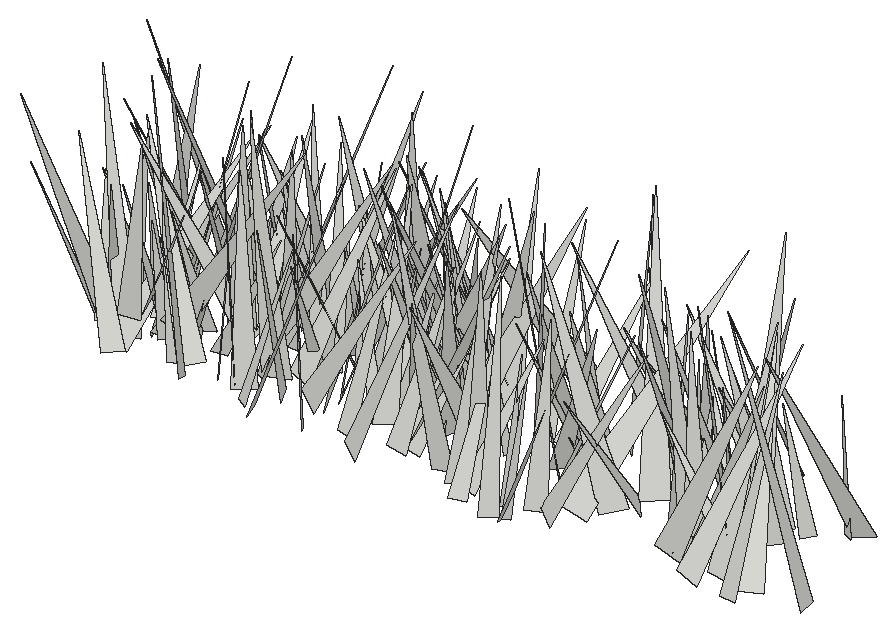
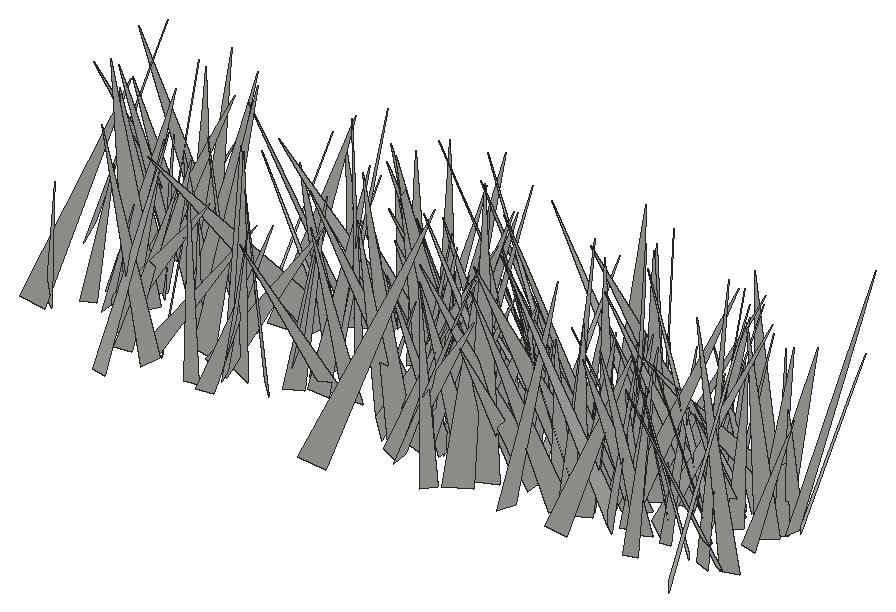
# SketchUp Ruby script. Lengths in inches.
U = 1.inch
M = Sketchup.active_model
def pt(a) = Geom::Point3d.new(a.map { |v| v * U })
def face(e, loops, mat)
  f = e.add_face(loops[0].map { |a| pt(a) })
  loops[1..].each { |l| e.add_face(l.map { |a| pt(a) }).erase! }
  f.material = f.back_material = mat if mat
  f
end
# faces: each face lists its corners as indices into pts; further lists are holes
def faces(e, pts, list, mat = nil) = list.each { |f| face(e, (f[0].is_a?(Array) ? f : [f]).map { |l| l.map { |i| pts[i] } }, mat) }
# xy, xz, yz: faces in a plane at the given z, y or x. An outline is a flat list of corners, or four numbers for a rectangle; further outlines are holes
def ring(l) = l.size == 4 ? [[l[0], l[1]], [l[2], l[1]], [l[2], l[3]], [l[0], l[3]]] : l.each_slice(2).to_a
def flat(e, list, mat, &to3) = list.each { |f| face(e, (f[0].is_a?(Array) ? f : [f]).map { |l| ring(l).map { |u, v| to3.(u, v) } }, mat) }
def xy(e, z, list, mat = nil) = flat(e, list, mat) { |x, y| [x, y, z] }
def xz(e, y, list, mat = nil) = flat(e, list, mat) { |x, z| [x, y, z] }
def yz(e, x, list, mat = nil) = flat(e, list, mat) { |y, z| [x, y, z] }
def lines(e, pts, list) = list.each { |a, b| e.add_line(pt(pts[a]), pt(pts[b])) }
# prism: a flat outline (further loops are holes) pulled along v
def prism(e, loops, v, mat = nil)
  f = face(e, loops, mat); d = Geom::Vector3d.new(v.map { |x| x * U })
  f.pushpull(f.normal.samedirection?(d) ? d.length : -d.length)
end
def box(e, o, s, mat = nil) = prism(e, [[o, [o[0] + s[0], o[1], o[2]], [o[0] + s[0], o[1] + s[1], o[2]], [o[0], o[1] + s[1], o[2]]]], [0, 0, s[2]], mat)
def at(x, y, z, deg = 0) = Geom::Transformation.translation(pt([x, y, z])) * Geom::Transformation.rotation(ORIGIN, Z_AXIS, deg.degrees)
def axes(o, x, y, z) = Geom::Transformation.new([*x, 0, *y, 0, *z, 0, *pt(o).to_a, 1])
def part(name) = M.definitions.add(name)
# library, detail: a bought-in or finely detailed component or shape, given as its bounding box
def library(name, o, s) = part(name).tap { |d| box(d.entities, o, s) }
def detail(e, o, s) = box(e.add_group.entities, o, s)
def put(e, d, t, mat = nil) = e.add_instance(d, t).tap { |i| i.material = mat if mat }
def group(e, t, mat = nil) = e.add_group.tap { |g| g.transformation = t; g.material = mat if mat }.entities
root = M.entities
c1 = part("fur_instance\#9")
p = [[0.8125,0,1.79],[0.67,-0.02,1.48],[0,-0.11,0],[0,0.11,0]]
faces(c1.entities,p,[[0,1,2,3]])
put(root,c1,axes([95.93,447.23,-27.1],[-3.80527,0.70423,0.62745],[0.3357,3.44844,-1.83447],[0.88144,1.72686,3.40746]))
put(root,c1,axes([97.41,448.625,-27.1],[3.70489,5.29932,0.63458],[5.07029,-3.25343,-2.43293],[1.66665,-1.88258,5.99082]))
put(root,c1,axes([95.1,446.8125,-27.1],[-5.93651,2.05948,0.4431],[1.83167,5.70073,-1.95618],[1.04056,1.71471,5.97135]))
put(root,c1,axes([96.62,448.84,-27.1],[-2.20726,4.7722,2.01563],[5.04733,2.47451,-0.33147],[1.16667,-1.67676,5.24748]))
put(root,c1,axes([78.89,450.2,-27.1],[-4.44854,-2.43941,1.67916],[-2.34276,4.75236,0.69742],[1.81157,0.15557,5.02532]))
put(root,c1,axes([100.51,452.55,-27.1],[-3.99829,-3.957,0.07334],[-3.50173,3.58563,2.55553],[1.84422,-1.77059,5.01133]))
put(root,c1,axes([90.21,449.16,-27.1],[-1.59145,-6.67923,2.98055],[-7.18236,0.85085,-1.92829],[-1.38185,3.26993,6.58988]))
put(root,c1,axes([68.83,449.93,-27.1],[3.92094,-4.8226,1.73149],[-5.06492,-3.97791,0.39007],[-0.77596,1.59628,6.20315]))
put(root,c1,axes([81.86,448.05,-27.1],[-4.19914,-2.372,1.71601],[-2.90919,3.71707,-1.98087],[0.32817,2.60017,4.39719]))
put(root,c1,axes([69.15,448.31,-27.1],[-3.00084,5.06154,0.45444],[5.0055,2.85272,1.2797],[-0.87785,-1.03611,5.74339]))
put(root,c1,axes([65.8125,451.81,-27.1],[-7.05336,-2.15617,1.71578],[-1.62887,7.06566,2.18314],[2.22256,-1.66441,7.04506]))
put(root,c1,axes([78.5625,447.95,-27.1],[6.55777,3.05775,0.67545],[3.00333,-6.58518,0.65252],[-0.88663,0.30968,7.20614]))
put(root,c1,axes([85.25,447.75,-27.1],[4.54632,6.46757,0.61256],[6.48609,-4.47646,-0.87508],[0.36794,-1.0028,7.85702]))
put(root,c1,axes([104.68,449.58,-27.1],[2.05152,-6.6713,2.37008],[-6.64568,-0.96384,3.03943],[2.44098,2.98279,6.28306]))
put(root,c1,axes([95.06,448.26,-27.1],[-3.85021,0.78609,0.9669],[0.45373,3.80886,-1.28983],[1.16059,1.11875,3.71193]))
put(root,c1,axes([74.96,449.76,-27.1],[2.81827,1.89164,1.24112],[2.11841,-2.90244,-0.38665],[-0.79437,-1.02901,3.37216]))
put(root,c1,axes([65.68,451.29,-27.1],[-3.97352,-3.33663,0.47318],[-3.25036,3.98768,0.8243],[0.89005,-0.33346,5.12275]))
put(root,c1,axes([75.72,450.125,-27.1],[4.83002,3.67653,3.08875],[4.26917,-5.29337,-0.3752],[-2.19806,-2.20219,6.05848]))
put(root,c1,axes([76.89,449.51,-27.1],[3.45962,-4.50001,2.91683],[-5.02174,-3.93643,-0.1168],[-1.88153,2.2319,5.67498]))
put(root,c1,axes([77.69,448.28,-27.1],[2.30646,3.84948,0.31393],[3.83736,-2.32546,0.32205],[-0.43787,-0.10267,4.47599]))
put(root,c1,axes([92.46,448.33,-27.1],[0.05703,4.78722,0.58826],[4.57544,0.13244,-1.52137],[1.52606,-0.57598,4.5394]))
put(root,c1,axes([91.9375,449.9,-27.1],[5.0258,-2.8928,2.35137],[-3.11716,-5.42578,-0.01254],[-2.04464,1.16127,5.79886]))
put(root,c1,axes([92.71,447.29,-27.1],[-4.05374,2.9207,0.15477],[2.65047,3.78022,-1.91631],[1.23673,1.47198,4.61422]))
put(root,c1,axes([108.58,450.4375,-27.1],[-4.58076,1.47717,0.18742],[1.47131,4.39705,1.30451],[-0.22897,-1.29786,4.63288]))
put(root,c1,axes([110.08,447.79,-27.1],[1.80185,5.93958,0.37976],[5.89361,-1.83593,0.75111],[-0.82954,-0.14229,6.16126]))
put(root,c1,axes([89.45,452.92,-27.1],[5.03177,-2.92165,1.14225],[-2.20313,-4.82824,-2.64459],[-2.23316,-1.81978,5.18275]))
put(root,c1,axes([113.78,449.7,-27.1],[-7.70081,-2.50661,0.76749],[-2.60656,7.57519,-1.4131],[0.27927,1.58364,7.97425]))
put(root,c1,axes([86.01,452.38,-27.1],[5.48383,-1.63022,0.30334],[-1.45467,-5.23263,-1.82362],[-0.79597,-1.66854,5.42259]))
put(root,c1,axes([80.25,450.53,-27.1],[3.77376,6.10396,1.49671],[5.76595,-2.66802,-3.65722],[2.50047,-3.05991,6.17449]))
put(root,c1,axes([72.33,449.4,-27.1],[-0.0394,4.36961,1.02441],[4.32756,-0.23455,1.1669],[-1.18959,-0.99797,4.2111]))
put(root,c1,axes([70.46,451.1,-27.1],[2.53184,-2.74895,1.13947],[-2.76231,-2.72751,-0.44237],[-1.1067,0.51894,3.71097]))
put(root,c1,axes([88.15,452.46,-27.1],[6.15158,-3.29467,0.71793],[-3.15743,-6.15236,-1.17953],[-1.18361,-0.7112,6.87789]))
put(root,c1,axes([69.88,451.81,-27.1],[-4.44345,-1.97155,1.25823],[-1.71315,4.58269,1.13072],[1.59225,-0.57131,4.72787]))
put(root,c1,axes([87,449.35,-27.1],[0.12132,5.40428,1.16344],[5.42728,0.10479,-1.05269],[1.05091,-1.16504,5.30215]))
put(root,c1,axes([105.55,450.54,-27.1],[-7.11208,1.53537,2.26223],[1.65379,7.4363,0.15223],[2.17716,-0.6331,7.27433]))
put(root,c1,axes([73.58,448.48,-27.1],[-7.24108,-2.76695,1.69952],[-3.23599,6.49389,-3.21487],[0.2698,3.62643,7.05364]))
put(root,c1,axes([105.69,450.78,-27.1],[3.10657,-5.20372,2.6425],[-5.63717,-3.45056,-0.16782],[-1.51121,2.17421,6.05816]))
put(root,c1,axes([83.98,449.01,-27.1],[1.01663,5.56132,0.68679],[5.60282,-1.02017,-0.03274],[-0.09106,-0.68151,5.65338]))
put(root,c1,axes([68.67,451.19,-27.1],[4.5818,0.64032,0.1617],[0.65902,-4.5067,-0.82732],[-0.04299,-0.84188,4.55176]))
put(root,c1,axes([107.08,448.19,-27.1],[1.06363,7.1406,0.14161],[6.98782,-1.01087,-1.51263],[1.47601,-0.35985,7.05914]))
put(root,c1,axes([105.9,450.67,-27.1],[5.04993,-3.13211,0.88061],[-3.25342,-4.87587,1.31476],[-0.02926,1.58216,5.79512]))
put(root,c1,axes([95.79,446.95,-27.1],[6.81061,4.1437,0.72104],[3.52808,-6.3754,3.31382],[-2.28972,2.50169,7.25074]))
put(root,c1,axes([66.07,452.39,-27.1],[4.73789,-1.18845,0.72275],[-0.9672,-4.65874,-1.32025],[-0.99966,-1.12521,4.70287]))
put(root,c1,axes([91.59,448.7,-27.1],[-6.63675,3.07759,1.929],[2.57186,6.8191,-2.03087],[2.56478,1.12578,7.02806]))
put(root,c1,axes([77.43,451.46,-27.1],[-2.10134,6.53759,3.4605],[7.38552,2.05442,0.60354],[0.41142,-3.48856,6.84043]))
put(root,c1,axes([81.06,451.06,-27.1],[7.00496,3.81978,0.96353],[3.93839,-6.83549,-1.53416],[-0.09034,-1.80938,7.82984]))
put(root,c1,axes([73.15,449.84,-27.1],[-5.62336,3.63446,0.06059],[3.63174,5.6129,0.37548],[-0.15301,-0.3482,6.6851]))
put(root,c1,axes([108.1,450.74,-27.1],[-5.99226,-3.56649,1.99916],[-3.93709,5.99,-1.11487],[1.10264,2.00593,6.88361]))
put(root,c1,axes([99.76,451.31,-27.1],[-4.16416,5.80884,2.0419],[6.1268,3.66414,2.07088],[-0.6118,-2.84317,6.84063]))
put(root,c1,axes([103.8,453.76,-27.1],[-0.44109,-6.89492,0.21564],[-6.89758,0.44393,0.08524],[0.09888,0.20974,6.90849]))
put(root,c1,axes([87.5,450.59,-27.1],[6.84085,-1.05323,0.60817],[-1.14548,-6.7472,1.19982],[-0.40871,1.28156,6.81667]))
put(root,c1,axes([108.29,449.29,-27.1],[1.00933,7.00307,0.82634],[7.04916,-1.02422,0.06983],[-0.18746,-0.80782,7.07509]))
put(root,c1,axes([87.49,449.76,-27.1],[-0.99691,5.86129,1.26655],[5.41282,1.43213,-2.36709],[2.58075,-0.73958,5.45394]))
put(root,c1,axes([105.18,451.03,-27.1],[2.53545,-3.02814,1.98338],[-3.53036,-2.60371,0.53779],[-0.80002,1.89288,3.91266]))
put(root,c1,axes([108.45,451.85,-27.1],[-2.5015,-6.23633,1.72664],[-6.18785,1.76379,-2.59425],[-1.89304,2.47545,6.19832]))
put(root,c1,axes([110.48,449.07,-27.1],[-3.69849,5.78351,0.10997],[5.76561,3.69627,-0.48502],[0.46777,0.16892,6.84781]))
put(root,c1,axes([87.125,453.27,-27.1],[-0.56263,-5.96411,0.83016],[-5.9756,0.45013,-0.816],[-0.74291,0.89616,5.93475]))
put(root,c1,axes([78.87,453.23,-27.1],[0.77798,-4.23548,0.16889],[-4.23878,-0.77834,0.00619],[-0.02442,0.16723,4.30633]))
put(root,c1,axes([84.37,451.11,-27.1],[-3.97928,1.73175,0.54979],[1.73454,4.01483,-0.09183],[0.54094,-0.13447,4.3388]))
put(root,c1,axes([95.91,451.54,-27.1],[5.05169,2.87341,0.23488],[2.86098,-4.93803,-1.1233],[0.35552,-1.09113,5.70213]))
put(root,c1,axes([73.53,451.65,-27.1],[3.09859,-2.8989,0.71648],[-2.92503,-2.73871,1.56906],[0.60101,1.61681,3.94246]))
put(root,c1,axes([95.61,454.26,-27.1],[-4.40501,-3.46188,0.56585],[-3.18391,4.32713,1.68747],[1.47225,-1.00011,5.34239]))
put(root,c1,axes([70.34,451.16,-27.1],[5.69226,-5.26322,0.96159],[-5.00885,-4.7486,3.65927],[1.88086,3.28288,6.8347]))
put(root,c1,axes([71.4,452.86,-27.1],[-5.49942,-3.45806,0.94275],[-3.51329,5.5426,-0.16378],[0.70973,0.64178,6.49422]))
put(root,c1,axes([74.0625,453.6875,-27.1],[-7.08449,-0.21202,0.14595],[-0.16992,6.87165,1.73429],[0.19334,-1.72965,6.8722]))
put(root,c1,axes([104.59,449.875,-27.1],[3.23969,5.31398,1.47982],[4.81259,-3.56155,2.25346],[-2.69577,0.02794,5.80137]))
put(root,c1,axes([95.23,452.43,-27.1],[-5.96506,-5.04673,2.13711],[-5.35643,6.03696,-0.69462],[1.15994,1.92465,7.7826]))
put(root,c1,axes([66.67,450.65,-27.1],[-4.24883,1.88722,0.42776],[1.75815,4.19597,-1.04876],[0.80838,0.79335,4.52927]))
put(root,c1,axes([80.23,454.59,-27.1],[-3.47678,-4.99975,0.07246],[-4.93171,3.44331,0.95532],[0.82523,-0.48669,6.01439]))
put(root,c1,axes([87.87,451.76,-27.1],[1.06055,3.50039,1.15885],[3.68372,-1.05849,-0.17402],[-0.16095,-1.16074,3.65339]))
put(root,c1,axes([79.46,452.22,-27.1],[1.72384,-3.5656,0.8716],[-3.29525,-1.07913,2.10276],[1.61693,1.60212,3.35612]))
put(root,c1,axes([71.69,453.13,-27.1],[0.72019,-3.80208,0.86926],[-3.795,-0.88705,-0.73566],[-0.89965,0.69817,3.79912]))
put(root,c1,axes([106.7,452.5,-27.1],[-3.07228,-3.20464,1.70758],[-3.41257,3.31254,0.07678],[1.24093,1.17551,4.43878]))
put(root,c1,axes([94.75,453.05,-27.1],[4.6953,-3.04636,0.27903],[-3.0591,-4.67738,0.40996],[-0.01004,0.49581,5.58194]))
put(root,c1,axes([68.43,453.28,-27.1],[3.6116,-2.54944,1.03868],[-2.46348,-3.75778,-0.65768],[-1.22872,0.0404,4.37159]))
put(root,c1,axes([68.17,450.66,-27.1],[-6.64184,2.29308,0.28161],[2.23011,6.58737,-1.04152],[0.60342,0.8944,6.94892]))
put(root,c1,axes([66.43,453.1,-27.1],[2.75053,-5.09352,1.52718],[-5.31748,-2.64324,0.76119],[-0.02665,1.70616,5.73847]))
put(root,c1,axes([86.78,452.53,-27.1],[-3.90024,1.94852,0.94584],[2.05782,3.9414,0.36592],[0.67579,-0.75618,4.3445]))
put(root,c1,axes([68.76,448.98,-27.1],[-3.50989,5.55769,0.51718],[4.45011,3.15505,-3.70364],[3.36927,1.62248,5.4305]))
put(root,c1,axes([103.18,453.01,-27.1],[-1.62958,-3.15436,1.09529],[-3.33909,1.53504,-0.54711],[-0.01197,1.22427,3.50802]))
put(root,c1,axes([73.36,453.7,-27.1],[4.72126,-4.87179,1.88096],[-5.03873,-4.91595,-0.08523],[-1.37242,1.28908,6.78361]))
put(root,c1,axes([75.08,453.34,-27.1],[4.55418,4.59674,3.34406],[5.23121,-5.06575,-0.16086],[-2.22422,-2.50228,6.46875]))
put(root,c1,axes([92.86,453.63,-27.1],[6.58164,2.52237,2.667],[2.99732,-6.85363,-0.91486],[-2.11926,-1.85972,6.9888]))
put(root,c1,axes([108.49,453.9,-27.1],[-3.08305,4.83073,2.80211],[5.58378,2.72141,1.452],[0.09585,-3.15451,5.54372]))
put(root,c1,axes([84.8,451.21,-27.1],[-5.4201,3.31702,1.28358],[3.06796,5.54385,-1.37151],[1.7994,0.53923,6.20476]))
put(root,c1,axes([69.67,450.875,-27.1],[3.36886,3.17868,0.5186],[2.75759,-3.23451,1.91201],[-1.66392,1.0752,4.2187]))
put(root,c1,axes([107.08,452.55,-27.1],[-4.22119,3.06488,0.48562],[3.10212,4.18863,0.52921],[0.07866,-0.71394,5.1896]))
put(root,c1,axes([85.35,454.27,-27.1],[4.73655,-6.32836,0.37656],[-6.13582,-4.45802,2.25891],[1.59428,1.644,7.57499]))
put(root,c1,axes([87.41,454.48,-27.1],[0.83878,-6.84447,1.51714],[-6.71971,-0.34936,2.13903],[1.99848,1.69801,6.55552]))
put(root,c1,axes([85.33,452.28,-27.1],[3.14685,5.37097,0.90824],[5.43729,-3.03382,-0.89816],[0.32882,-1.23429,6.15981]))
put(root,c1,axes([85.1,455.28,-27.1],[-7.14717,-1.7401,1.8273],[-1.33254,7.26397,1.70532],[2.14274,-1.28679,7.15555]))
put(root,c1,axes([88.83,454.86,-27.1],[2.63547,-2.52355,0.88422],[-2.24578,-2.7628,-1.19134],[-1.45143,-0.30736,3.44888]))
put(root,c1,axes([94.06,455.55,-27.1],[0.0355,-6.28923,0.69696],[-6.32457,-0.05728,-0.19472],[-0.19984,0.69551,6.28631]))
put(root,c1,axes([89.85,452.54,-27.1],[-6.30755,-1.0303,0.95825],[-1.23667,6.15876,-1.51833],[0.67114,1.66527,6.20817]))
put(root,c1,axes([75.9,454.39,-27.1],[0.59547,-6.22896,1.95156],[-6.50827,-0.41619,0.65745],[0.50087,1.99748,6.22272]))
put(root,c1,axes([91.82,452.55,-27.1],[-4.16837,-0.36819,0.02902],[-0.35612,3.91965,-1.4217],[-0.09791,1.41863,3.93569]))
put(root,c1,axes([66.56,454.52,-27.1],[-0.08918,-3.86635,0.81214],[-3.84672,-0.10019,-0.89937],[-0.90053,0.81086,3.76135]))
put(root,c1,axes([76.6875,451.05,-27.1],[3.68113,4.53912,0.36663],[4.24955,-3.59341,1.82137],[-1.63686,0.87892,5.5531]))
put(root,c1,axes([78.4375,452.1,-27.1],[1.11802,6.55656,0.88639],[6.4324,-0.86675,-1.70208],[1.54866,-1.13332,6.42972]))
put(root,c1,axes([81.57,451.53,-27.1],[4.34106,2.99141,0.28027],[2.79242,-4.19877,1.56351],[-1.10882,1.13738,5.03476]))
put(root,c1,axes([101.26,456,-27.1],[-1.0754,-7.3325,1.08617],[-7.40599,1.10888,0.15329],[0.31086,1.05196,7.40935]))
put(root,c1,axes([75.03,454.46,-27.1],[4.40787,6.56573,1.54887],[6.23945,-3.26461,-3.91775],[2.5646,-3.34225,6.86945]))
put(root,c1,axes([71.49,455.91,-27.1],[-3.69679,-5.87263,0.02895],[-5.78236,3.6339,-1.23044],[-1.02613,0.67962,6.82936]))
put(root,c1,axes([84.16,453.32,-27.1],[3.26385,-1.40609,1.47007],[-1.85279,-3.20219,1.05074],[-0.83985,1.59994,3.39496]))
put(root,c1,axes([83.07,453.73,-27.1],[4.24313,0.45781,1.20359],[0.34307,-4.39664,0.46288],[-1.24117,0.34981,4.24258]))
put(root,c1,axes([81.36,451.83,-27.1],[4.43621,4.25023,1.48293],[3.65379,-4.61591,2.29927],[-2.62932,0.75659,5.69717]))
put(root,c1,axes([69.42,453.87,-27.1],[6.44327,3.68852,1.42181],[3.82977,-6.4983,-0.49739],[-0.97955,-1.14429,7.40767]))
put(root,c1,axes([76.3,452.3,-27.1],[-6.09623,-2.24198,1.5344],[-2.70516,5.35755,-2.91953],[0.25098,3.28863,5.80232]))
put(root,c1,axes([68.91,452.54,-27.1],[-2.94733,3.27814,0.42411],[3.06608,2.92358,-1.29021],[1.23501,0.56503,4.21525]))
put(root,c1,axes([95.22,456.09,-27.1],[3.85472,-3.45884,0.89823],[-3.26491,-3.94586,-1.18314],[-1.45282,-0.30973,5.04209]))
put(root,c1,axes([79.3,453.91,-27.1],[-0.34348,3.88251,1.09091],[4.02925,0.37671,-0.07204],[0.17064,-1.07988,3.89701]))
put(root,c1,axes([74.78,455.08,-27.1],[2.18952,-4.24382,2.13551],[-4.35668,-2.73133,-0.96101],[-1.89466,1.3763,4.67766]))
put(root,c1,axes([98.12,449.93,-27.1],[-4.06981,7.2471,0.38585],[5.9474,3.58401,-4.58433],[4.15906,1.9665,6.9331]))
put(root,c1,axes([86.23,457.1,-27.1],[-1.07248,-7.00957,0.36815],[-6.96342,1.01561,-0.94825],[-0.88342,0.50425,7.02746]))
put(root,c1,axes([70.2,456.81,-27.1],[-1.799,-4.93024,0.4482],[-4.7112,1.85147,1.45641],[1.52075,-0.09654,5.04207]))
put(root,c1,axes([73.57,455.84,-27.1],[-3.74944,-6.99723,1.04952],[-6.92154,3.38084,-2.18706],[-1.468,1.93125,7.63127]))
put(root,c1,axes([111.46,457.32,-27.1],[1.05272,-6.58483,0.46236],[-6.33643,-1.13928,-1.79827],[-1.85027,0.15508,6.42141]))
put(root,c1,axes([86.12,454.78,-27.1],[3.3067,2.95122,2.18217],[3.23124,-3.73382,0.15332],[-1.74087,-1.32466,4.4295]))
put(root,c1,axes([83.76,454.94,-27.1],[-3.5373,3.73043,1.14853],[3.88761,3.22863,1.48666],[-0.34887,-1.84596,4.92122]))
put(root,c1,axes([82.12,456.38,-27.1],[3.81403,-1.87609,0.65313],[-1.66249,-3.78837,-1.17367],[-1.0874,-0.78844,4.08523]))
put(root,c1,axes([71.63,451.79,-27.1],[6.96857,3.90701,1.2479],[3.36407,-6.85211,2.66731],[-2.34628,1.77954,7.53068]))
put(root,c1,axes([109.25,455.49,-27.1],[2.35364,-2.97334,1.61897],[-3.0072,-2.74184,-0.66374],[-1.55518,0.80187,3.73361]))
put(root,c1,axes([76.64,456.96,-27.1],[6.75782,0.35235,2.65885],[1.16075,-6.88187,-2.03823],[-2.41791,-2.31896,6.45275]))
put(root,c1,axes([80.28,455.16,-27.1],[3.33409,-2.8819,1.80128],[-3.12207,-3.59416,0.02846],[-1.34262,1.20116,4.40689]))
put(root,c1,axes([72.57,456.74,-27.1],[2.27929,-4.31761,0.37807],[-4.29346,-2.30768,-0.46977],[-0.59235,0.11282,4.85966]))
put(root,c1,axes([105.82,456.99,-27.1],[1.37303,-5.10418,0.31363],[-5.09334,-1.39399,-0.38851],[-0.45708,0.20095,5.27134]))
put(root,c1,axes([79.76,455.91,-27.1],[-0.47471,-3.8388,0.84095],[-3.92781,0.49062,0.02236],[0.12592,0.83177,3.86797]))
put(root,c1,axes([102.78,454.45,-27.1],[1.15906,3.62365,1.13013],[3.60388,-1.42153,0.86183],[-1.19166,-0.77453,3.7056]))
put(root,c1,axes([83.41,452.66,-27.1],[6.6915,4.26773,1.20587],[3.94044,-6.72308,1.92792],[-2.03484,1.01512,7.69888]))
put(root,c1,axes([86.33,456.68,-27.1],[-4.22717,-2.44585,1.01456],[-2.28976,4.33627,0.91336],[1.32985,-0.3083,4.79759]))
put(root,c1,axes([67.24,457.44,-27.1],[-3.46246,-6.72611,1.90114],[-6.59046,3.84836,1.61233],[2.32826,0.89059,7.39118]))
put(root,c1,axes([75.32,456.73,-27.1],[3.88583,-1.17381,1.38743],[-0.79486,-4.04284,-1.19419],[-1.63432,-0.82466,3.87962]))
put(root,c1,axes([72.09,456.46,-27.1],[1.922,-3.18961,0.22781],[-3.1707,-1.86642,0.61867],[0.41494,0.51232,3.67219]))
put(root,c1,axes([106.47,454.43,-27.1],[5.95771,-4.00613,4.25574],[-5.13988,-6.48421,1.09155],[-2.78246,3.40011,7.09591]))
put(root,c1,axes([87.35,457.0625,-27.1],[2.07111,-6.85146,1.31632],[-6.80663,-1.68294,1.94991],[1.53132,1.78604,6.88693]))
put(root,c1,axes([68.85,454.81,-27.1],[3.76051,3.97563,0.83952],[4.01253,-3.81366,0.08642],[-0.64034,-0.54974,5.47171]))
put(root,c1,axes([108.1,455.35,-27.1],[-4.0966,0.35691,0.30901],[0.31396,4.07547,-0.54495],[0.35257,0.51784,4.07585]))
put(root,c1,axes([103.57,457.44,-27.1],[-0.91918,-4.72146,0.08029],[-4.18667,0.777,-2.23865],[-2.18412,0.49761,4.25741]))
put(root,c1,axes([89.28,456.5,-27.1],[-4.75874,-5.64309,0.42264],[-5.39038,4.3522,-2.58279],[-1.72245,1.97043,6.91515]))
put(root,c1,axes([96.03,455.1,-27.1],[-5.27526,-0.92635,0.94955],[-1.13263,5.17215,-1.24665],[0.69057,1.40673,5.20887]))
put(root,c1,axes([85.59,455.97,-27.1],[-3.98273,-4.40716,0.90523],[-4.3967,3.55588,-2.0321],[-0.95477,2.0093,5.58174]))
put(root,c1,axes([75.32,457.24,-27.1],[3.57581,-3.48366,1.446],[-3.33217,-3.85124,-1.03819],[-1.76733,0.21279,4.88308]))
put(root,c1,axes([104.77,458.24,-27.1],[2.5877,-3.76016,0.15432],[-3.53923,-2.49522,-1.45139],[-1.27925,-0.70276,4.32764]))
put(root,c1,axes([100.7,453.56,-27.1],[-7.32021,3.8589,0.48336],[3.73123,7.2592,-1.44642],[1.09666,1.05977,8.14767]))
put(root,c1,axes([107.57,455.1,-27.1],[-2.18408,5.95276,0.46734],[5.01759,1.55993,3.57972],[-3.2369,-1.59851,5.23366]))
put(root,c1,axes([86.68,456.46,-27.1],[0.19192,-5.71021,2.24229],[-6.02696,-0.59408,-0.99702],[-1.14462,2.17066,5.62577]))
put(root,c1,axes([71.11,455.25,-27.1],[3.02903,2.92229,1.12241],[2.89072,-3.2105,0.55771],[-1.2014,-0.35704,4.17178]))
put(root,c1,axes([87.36,455.18,-27.1],[0.42432,7.03314,2.02201],[6.63788,0.48281,-3.07232],[3.08094,-2.00885,6.34082]))
put(root,c1,axes([85,456.33,-27.1],[4.99939,-0.31235,0.02616],[-0.31267,-4.999,0.06629],[-0.02197,0.06779,5.0087]))
put(root,c1,axes([76.66,456.02,-27.1],[4.45392,4.12687,0.87812],[4.21021,-4.26347,-1.31776],[0.27618,-1.55927,5.92722]))
put(root,c1,axes([81.53,457.59,-27.1],[2.47243,-7.62212,2.09201],[-7.90302,-2.41845,0.52868],[-0.12434,2.1542,7.99563]))
put(root,c1,axes([65.71,457.07,-27.1],[-0.42435,-6.57592,2.54627],[-6.78158,1.0798,1.65847],[1.93298,2.34469,6.37748]))
put(root,c1,axes([82.26,458.83,-27.1],[5.27875,-5.42072,0.96709],[-5.29735,-5.36505,-1.15714],[-1.50251,-0.12916,7.47733]))
put(root,c1,axes([77.51,454.89,-27.1],[0.02975,6.47261,1.15989],[6.34372,-0.33363,1.69906],[-1.73125,-1.11127,6.2457]))
put(root,c1,axes([78.87,453.2,-27.1],[7.42059,-0.17453,3.00871],[-1.57677,-7.03899,3.48057],[-2.56838,3.81708,6.55601]))
put(root,c1,axes([92.18,455.05,-27.1],[0.04484,6.03011,0.93276],[6.10111,-0.02998,-0.09948],[0.09373,-0.93336,6.02946]))
put(root,c1,axes([78.27,455.24,-27.1],[-5.05186,2.37101,0.85511],[2.22237,5.09377,-0.9944],[1.18912,0.55319,5.49128]))
put(root,c1,axes([99.77,456.79,-27.1],[-2.20634,6.02099,1.75888],[5.48729,0.94934,3.63349],[-3.03901,-2.65713,5.28374]))
put(root,c1,axes([73.49,457.31,-27.1],[-2.97615,-4.05495,1.48787],[-4.26463,3.04523,-0.23114],[0.68511,1.34083,5.02461]))
put(root,c1,axes([79.25,455.89,-27.1],[6.564,-1.73993,0.0582],[-1.67851,-6.26496,2.01239],[0.46191,1.95953,6.48565]))
put(root,c1,axes([68.47,457.03,-27.1],[4.49917,3.28934,0.87918],[3.40387,-4.3112,-1.28935],[0.07989,-1.55853,5.42216]))
put(root,c1,axes([84.3,455.6,-27.1],[-1.65909,5.33475,1.21269],[5.33342,1.85943,-0.88312],[1.21852,-0.87506,5.51654]))
put(root,c1,axes([70.81,458.9,-27.1],[-0.56005,-4.94681,0.27227],[-4.82604,0.60667,1.09544],[1.12,0.14049,4.85639]))
put(root,c1,axes([98.72,459.04,-27.1],[3.46257,-3.0651,1.27719],[-2.41097,-3.5895,-2.07802],[-2.28326,-0.85797,4.13111]))
put(root,c1,axes([89.42,455.58,-27.1],[-0.62472,6.74476,1.37593],[6.88336,0.62526,0.06028],[0.06565,-1.37569,6.77336]))
put(root,c1,axes([71.62,456.78,-27.1],[0.44835,5.06558,1.88586],[5.29017,-0.02286,-1.19629],[1.10933,-1.93829,4.94267]))
put(root,c1,axes([93.52,454.99,-27.1],[-0.37436,5.47936,0.25355],[5.20879,0.43477,-1.70506],[1.71934,-0.12411,5.22075]))
put(root,c1,axes([110.82,456.79,-27.1],[1.66971,3.21733,1.57549],[3.35444,-2.01427,0.55833],[-1.25742,-1.10127,3.58153]))
put(root,c1,axes([73.21,455.02,-27.1],[-2.73527,5.15415,0.70761],[4.98067,2.82527,-1.3261],[1.50298,0.0175,5.68229]))
put(root,c1,axes([98.45,456.56,-27.1],[1.87849,6.8023,2.53671],[7.02619,-2.36292,1.13321],[-1.82724,-2.09291,6.96533]))
put(root,c1,axes([102.99,457.16,-27.1],[-3.64875,-2.02244,1.121],[-2.25149,3.58457,-0.86132],[0.52696,1.3118,4.08188]))
put(root,c1,axes([87.96,456.22,-27.1],[-2.08516,6.03207,0.25096],[5.29839,1.7011,3.1353],[-2.89412,-1.23172,5.5591]))
put(root,c1,axes([86.47,458.33,-27.1],[-6.23663,-1.3966,0.55844],[-1.37103,6.25805,0.33911],[0.61857,-0.21031,6.38209]))
put(root,c1,axes([76.94,457.11,-27.1],[6.19791,-1.23637,0.25272],[-1.26158,-6.10069,1.0939],[-0.02993,1.12232,6.22464]))
put(root,c1,axes([75.44,459.25,-27.1],[1.50286,-5.49819,1.33251],[-5.18917,-1.88889,-1.94134],[-2.25347,0.68284,5.35909]))
put(root,c1,axes([81.19,455.04,-27.1],[-4.89219,1.92037,1.37183],[1.09822,4.64707,-2.5888],[2.08893,2.05431,4.57377]))
put(root,c1,axes([87.12,458.32,-27.1],[-0.99125,-4.30354,0.98962],[-4.28593,0.69339,-1.27766],[-1.06332,1.21702,4.22737]))
put(root,c1,axes([89.71,461.48,-27.1],[4.2838,-6.03866,0.74714],[-5.20831,-4.11147,-3.36808],[-3.14598,-1.41597,6.59337]))
put(root,c1,axes([98.96,457.02,-27.1],[-4.99068,-1.45127,1.21381],[-1.71677,4.91279,-1.18474],[0.79513,1.49823,5.06058]))
put(root,c1,axes([78.98,458.875,-27.1],[-6.42976,0.15301,2.02637],[0.5172,6.6259,1.14077],[1.96522,-1.24316,6.3296]))
put(root,c1,axes([99.82,458.8,-27.1],[-0.19463,-4.95849,1.24268],[-5.00803,0.4343,0.94858],[1.02496,1.18047,4.8708]))
put(root,c1,axes([67.26,460.17,-27.1],[-6.10704,-5.17922,1.29191],[-4.99805,6.23748,1.37932],[1.87424,-0.24245,7.88782]))
put(root,c1,axes([66.34,457.08,-27.1],[3.26284,4.45559,0.15103],[4.26787,-3.06768,-1.7017],[1.28856,-1.1217,5.25381]))
put(root,c1,axes([96.39,456.85,-27.1],[4.10758,4.73433,2.04961],[4.7509,-4.49256,0.85604],[-2.01089,-0.9434,6.20913]))
put(root,c1,axes([102.83,458.39,-27.1],[6.50661,-0.43072,0.76621],[-0.39332,-6.54513,-0.33931],[-0.78607,-0.29036,6.51202]))
put(root,c1,axes([74.08,456.22,-27.1],[7.5502,3.19495,0.69372],[3.12341,-7.56468,0.84526],[-0.96605,0.51231,8.15468]))
put(root,c1,axes([83.39,459.77,-27.1],[5.22724,-1.35677,0.09683],[-1.28473,-5.05093,-1.4184],[-0.44684,-1.34966,5.21086]))
put(root,c1,axes([104.26,460.88,-27.1],[-2.87377,-5.9267,0.11201],[-5.79461,2.83495,1.33509],[1.24935,-0.48389,6.44995]))
